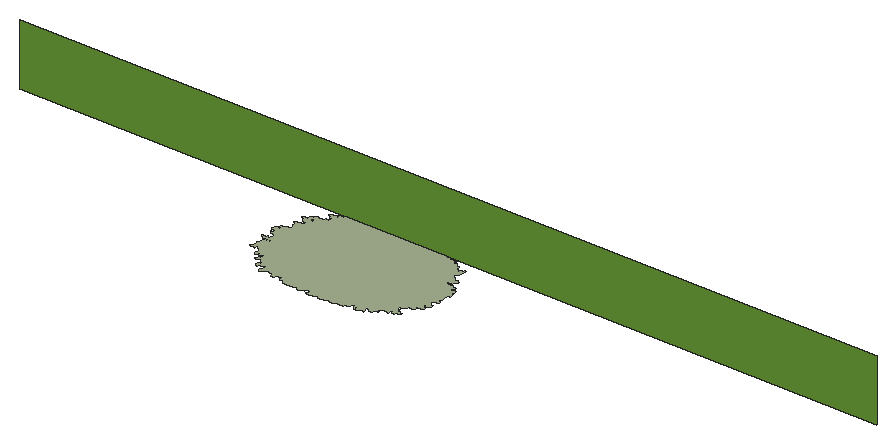
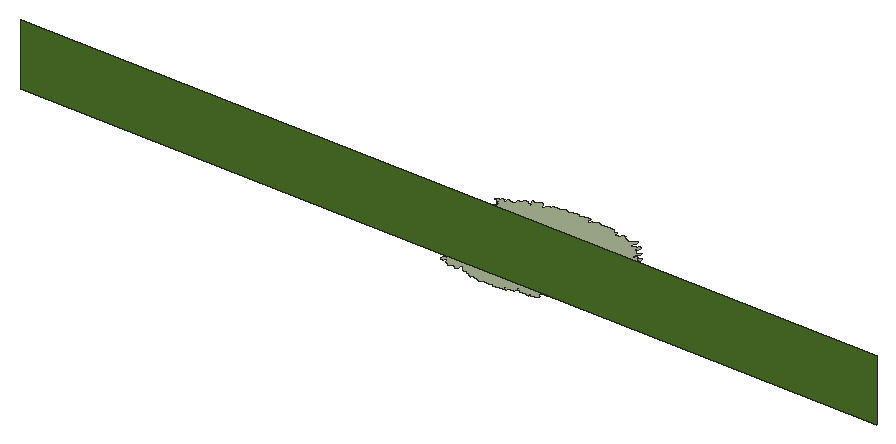
# SketchUp Ruby script. Lengths in inches.
U = 1.inch
M = Sketchup.active_model
def pt(a) = Geom::Point3d.new(a.map { |v| v * U })
def face(e, loops, mat)
  f = e.add_face(loops[0].map { |a| pt(a) })
  loops[1..].each { |l| e.add_face(l.map { |a| pt(a) }).erase! }
  f.material = f.back_material = mat if mat
  f
end
# faces: each face lists its corners as indices into pts; further lists are holes
def faces(e, pts, list, mat = nil) = list.each { |f| face(e, (f[0].is_a?(Array) ? f : [f]).map { |l| l.map { |i| pts[i] } }, mat) }
# xy, xz, yz: faces in a plane at the given z, y or x. An outline is a flat list of corners, or four numbers for a rectangle; further outlines are holes
def ring(l) = l.size == 4 ? [[l[0], l[1]], [l[2], l[1]], [l[2], l[3]], [l[0], l[3]]] : l.each_slice(2).to_a
def flat(e, list, mat, &to3) = list.each { |f| face(e, (f[0].is_a?(Array) ? f : [f]).map { |l| ring(l).map { |u, v| to3.(u, v) } }, mat) }
def xy(e, z, list, mat = nil) = flat(e, list, mat) { |x, y| [x, y, z] }
def xz(e, y, list, mat = nil) = flat(e, list, mat) { |x, z| [x, y, z] }
def yz(e, x, list, mat = nil) = flat(e, list, mat) { |y, z| [x, y, z] }
def lines(e, pts, list) = list.each { |a, b| e.add_line(pt(pts[a]), pt(pts[b])) }
# prism: a flat outline (further loops are holes) pulled along v
def prism(e, loops, v, mat = nil)
  f = face(e, loops, mat); d = Geom::Vector3d.new(v.map { |x| x * U })
  f.pushpull(f.normal.samedirection?(d) ? d.length : -d.length)
end
def box(e, o, s, mat = nil) = prism(e, [[o, [o[0] + s[0], o[1], o[2]], [o[0] + s[0], o[1] + s[1], o[2]], [o[0], o[1] + s[1], o[2]]]], [0, 0, s[2]], mat)
def at(x, y, z, deg = 0) = Geom::Transformation.translation(pt([x, y, z])) * Geom::Transformation.rotation(ORIGIN, Z_AXIS, deg.degrees)
def axes(o, x, y, z) = Geom::Transformation.new([*x, 0, *y, 0, *z, 0, *pt(o).to_a, 1])
def part(name) = M.definitions.add(name)
# library, detail: a bought-in or finely detailed component or shape, given as its bounding box
def library(name, o, s) = part(name).tap { |d| box(d.entities, o, s) }
def detail(e, o, s) = box(e.add_group.entities, o, s)
def put(e, d, t, mat = nil) = e.add_instance(d, t).tap { |i| i.material = mat if mat }
def group(e, t, mat = nil) = e.add_group.tap { |g| g.transformation = t; g.material = mat if mat }.entities
root = M.entities
M.materials.add("Boxwoodplan").color = [166, 177, 144]
M.materials.add("[Grass Dark Green]").color = [106, 157, 55]
xy(root,9.058,[[[87.354,67.129,87.243,67.133,87.148,67.159,87.092,67.215,87.091,67.317,87.117,67.382,87.18,67.445,87.229,67.509,87.288,67.606,87.101,67.635,87.011,67.644,87.031,67.732,87.117,67.79,87.148,67.8,87.143,67.846,87.054,67.877,86.938,67.837,86.841,67.706,86.699,67.551,86.538,67.464,86.432,67.441,86.372,67.416,86.356,67.373,86.211,67.281,86.018,67.251,85.929,67.26,85.848,67.306,85.848,67.328,85.894,67.359,85.984,67.437,86.053,67.483,85.963,67.498,85.851,67.48,85.731,67.436,85.537,67.454,85.44,67.447,85.314,67.403,85.113,67.356,85.024,67.349,84.986,67.443,84.978,67.465,84.911,67.473,84.822,67.454,84.654,67.336,84.454,67.328,84.224,67.353,84.057,67.446,83.915,67.61,84.098,67.702,83.999,67.756,83.863,67.772,83.737,67.749,83.664,67.697,83.584,67.672,83.468,67.738,83.426,67.806,83.513,67.847,83.54,67.907,83.545,67.957,83.504,68.009,83.431,68.085,83.346,68.117,83.259,68.064,83.192,68.038,83.136,68.08,83.12,68.103,83.096,68.121,83.066,68.111,82.987,68.058,82.915,68.01,82.839,67.923,82.828,67.79,82.756,67.749,82.706,67.723,82.646,67.725,82.547,67.746,82.461,67.793,82.417,67.861,82.408,67.951,82.417,68.018,82.43,68.04,82.411,68.08,82.198,68.1,82.266,68.135,82.239,68.136,82.147,68.13,81.977,68.146,81.9,68.173,81.883,68.206,81.897,68.224,82.023,68.314,82.02,68.371,81.936,68.393,81.776,68.39,81.646,68.319,81.548,68.233,81.474,68.199,81.426,68.172,81.425,68.154,81.462,68.101,81.446,68.046,81.375,68.081,81.312,68.121,81.251,68.072,81.228,68.017,81.197,67.904,81.149,67.855,81.076,67.822,80.985,67.816,80.915,67.841,80.897,67.874,80.904,67.892,80.925,67.932,80.947,67.991,80.916,68.048,80.815,68.149,80.929,68.229,80.99,68.269,81.069,68.285,81.137,68.315,81.192,68.37,81.276,68.476,81.205,68.503,81.125,68.511,80.993,68.53,80.954,68.565,80.962,68.584,81.036,68.62,81.198,68.657,81.241,68.709,81.236,68.748,81.21,68.764,81.06,68.711,81.014,68.732,81.015,68.752,81.037,68.814,80.876,68.825,80.796,68.833,80.742,68.826,80.734,68.806,80.718,68.71,80.703,68.642,80.662,68.591,80.615,68.578,80.595,68.594,80.536,68.639,80.492,68.757,80.452,68.783,80.425,68.784,80.372,68.777,80.365,68.757,80.363,68.641,80.308,68.523,80.248,68.449,80.168,68.419,80.089,68.422,80.042,68.448,80.009,68.506,80.01,68.564,80.063,68.677,80.177,68.784,80.198,68.803,80.184,68.823,80.158,68.829,80.077,68.847,79.997,68.86,79.97,68.875,79.976,68.895,79.997,68.914,80.145,68.982,80.307,69.005,80.349,69.108,80.323,69.169,80.276,69.191,80.248,69.187,80.085,69.168,80.045,69.2,80.051,69.22,80.079,69.279,80.236,69.334,80.408,69.403,80.457,69.442,80.443,69.463,80.347,69.436,80.175,69.417,80.031,69.372,79.942,69.386,79.915,69.392,79.922,69.412,79.942,69.426,79.997,69.47,79.97,69.507,79.942,69.503,79.86,69.511,79.805,69.56,79.791,69.601,79.763,69.597,79.681,69.575,79.524,69.489,79.374,69.413,79.3,69.38,79.245,69.392,79.258,69.412,79.278,69.452,79.304,69.469,79.329,69.55,79.378,69.65,79.41,69.759,79.461,69.812,79.535,69.852,79.579,69.972,79.601,70.112,79.62,70.227,79.616,70.285,79.571,70.321,79.491,70.335,79.404,70.335,79.331,70.31,79.321,70.245,79.321,70.184,79.288,70.124,79.2,70.087,79.144,70.096,79.105,70.155,79.095,70.216,79.069,70.337,79.063,70.4,79.023,70.453,78.995,70.475,78.958,70.491,78.899,70.479,78.864,70.46,78.863,70.428,78.855,70.366,78.857,70.229,78.882,70.167,78.874,70.103,78.824,70.038,78.775,70.01,78.737,69.998,78.7,70.003,78.658,70.011,78.64,70.039,78.636,70.166,78.657,70.223,78.702,70.276,78.718,70.306,78.709,70.334,78.652,70.34,78.571,70.346,78.533,70.362,78.51,70.39,78.507,70.453,78.523,70.483,78.557,70.499,78.73,70.472,78.808,70.497,78.858,70.526,78.918,70.573,78.932,70.636,78.909,70.662,78.865,70.664,78.787,70.67,78.695,70.681,78.594,70.717,78.576,70.746,78.581,70.76,78.601,70.763,78.66,70.775,78.836,70.761,78.925,70.787,78.938,70.844,78.912,70.907,78.84,70.946,78.761,70.953,78.647,70.946,78.548,70.921,78.464,70.939,78.46,70.968,78.481,70.997,78.527,71.054,78.594,71.11,78.647,71.19,78.638,71.224,78.594,71.241,78.529,71.24,78.411,71.14,78.371,71.141,78.337,71.161,78.358,71.22,78.375,71.287,78.331,71.35,78.291,71.366,78.271,71.367,78.266,71.352,78.27,71.306,78.267,71.164,78.226,71.102,78.186,71.108,78.152,71.131,78.054,71.262,78.029,71.327,78.005,71.355,77.989,71.344,77.934,71.293,77.899,71.234,77.918,71.103,77.923,71.037,77.903,70.971,77.854,70.962,77.819,70.978,77.809,71.023,77.829,71.155,77.839,71.233,77.839,71.27,77.824,71.282,77.809,71.272,77.729,71.237,77.69,71.183,77.68,71.12,77.641,71.077,77.504,70.987,77.465,70.977,77.42,70.986,77.341,71.026,77.32,71.056,77.324,71.089,77.357,71.151,77.455,71.237,77.544,71.263,77.634,71.263,77.729,71.267,77.669,71.318,77.517,71.404,77.501,71.466,77.554,71.503,77.645,71.573,77.764,71.635,77.883,71.709,77.918,71.723,77.944,71.746,77.971,71.789,77.974,71.882,78.006,72.003,78.007,72.065,77.986,72.086,77.965,72.095,77.902,72.109,77.868,72.104,77.865,72.088,77.876,71.996,77.835,71.934,77.787,71.899,77.709,71.871,77.638,71.858,77.478,71.833,77.443,71.839,77.429,71.853,77.43,71.86,77.438,71.901,77.455,71.947,77.497,71.995,77.567,72.042,77.625,72.063,77.684,72.065,77.722,72.068,77.742,72.075,77.765,72.096,77.761,72.121,77.706,72.151,77.638,72.207,77.606,72.264,77.602,72.331,77.615,72.382,77.668,72.426,77.694,72.432,77.705,72.425,77.724,72.411,77.767,72.35,77.816,72.304,77.945,72.226,78.018,72.192,78.054,72.177,78.074,72.184,78.098,72.206,78.104,72.222,78.116,72.263,78.1,72.32,78.058,72.366,78.025,72.389,77.992,72.401,77.932,72.401,77.858,72.404,77.814,72.446,77.728,72.519,77.67,72.569,77.631,72.617,77.631,72.646,77.655,72.671,77.712,72.698,77.747,72.703,77.788,72.7,77.848,72.679,77.909,72.677,77.945,72.684,77.98,72.726,78.028,72.757,78.088,72.764,78.159,72.764,78.3125,72.771,78.453,72.792,78.485,72.808,78.486,72.826,78.48,72.868,78.469,72.913,78.48,72.957,78.51,73.06,78.496,73.083,78.474,73.097,78.417,73.126,78.363,73.164,78.291,73.192,78.218,73.195,78.167,73.184,78.146,73.17,78.121,73.119,78.126,73.098,78.138,73.093,78.161,73.088,78.312,73.076,78.338,73.071,78.344,73.0625,78.334,73.046,78.295,73.007,78.249,72.964,78.185,72.928,78.123,72.884,78.05,72.849,78.013,72.852,77.994,72.863,77.968,72.9,77.961,72.995,77.944,73.02,77.962,73.034,77.969,73.077,77.963,73.088,77.951,73.088,77.937,73.087,77.911,73.083,77.878,73.076,77.861,73.065,77.78,72.97,77.748,72.915,77.717,72.892,77.694,72.895,77.668,72.916,77.659,72.932,77.653,72.973,77.681,73.057,77.687,73.102,77.678,73.13,77.657,73.137,77.619,73.128,77.599,73.114,77.553,73.064,77.432,72.957,77.395,72.932,77.37,72.927,77.332,72.935,77.32,72.951,77.412,73.057,77.474,73.102,77.488,73.129,77.488,73.145,77.479,73.152,77.467,73.148,77.453,73.143,77.421,73.131,77.338,73.108,77.17,73.089,77.097,73.096,77.05,73.121,77.028,73.149,77.027,73.165,77.044,73.217,77.091,73.264,77.152,73.281,77.222,73.284,77.297,73.266,77.424,73.223,77.51,73.197,77.522,73.201,77.522,73.209,77.521,73.22,77.512,73.239,77.488,73.287,77.486,73.342,77.494,73.407,77.505,73.437,77.523,73.45,77.571,73.413,77.611,73.363,77.638,73.317,77.647,73.255,77.66,73.204,77.674,73.176,77.698,73.175,77.832,73.157,77.905,73.144,77.94,73.14,77.958,73.154,77.974,73.202,77.918,73.244,77.86,73.309,77.842,73.335,77.842,73.352,77.876,73.46,77.906,73.483,77.934,73.489,77.948,73.477,77.957,73.459,77.986,73.414,77.998,73.39,78.01,73.391,78.031,73.404,78.111,73.482,78.127,73.528,78.129,73.579,78.115,73.611,78.094,73.623,78.03,73.646,77.991,73.666,77.982,73.687,77.998,73.736,78.054,73.773,78.089,73.795,78.102,73.816,78.109,73.869,78.108,73.916,78.012,73.992,77.869,74.014,77.806,74.031,77.772,74.013,77.743,74.014,77.674,74.031,77.655,74.058,77.665,74.082,77.791,74.185,77.784,74.217,77.762,74.233,77.718,74.225,77.689,74.216,77.563,74.154,77.523,74.107,77.473,74.063,77.404,74.049,77.376,74.05,77.329,74.102,77.357,74.126,77.375,74.165,77.407,74.188,77.5,74.22,77.545,74.25,77.535,74.281,77.522,74.283,77.512,74.276,77.486,74.27,77.446,74.273,77.311,74.284,77.165,74.3125,77.141,74.327,77.146,74.347,77.171,74.375,77.384,74.435,77.448,74.434,77.508,74.419,77.569,74.391,77.595,74.393,77.602,74.403,77.651,74.48,77.674,74.495,77.681,74.515,77.68,74.557,77.68,74.583,77.67,74.593,77.656,74.591,77.599,74.591,77.541,74.585,77.494,74.568,77.47,74.576,77.45,74.596,77.425,74.63,77.405,74.718,77.415,74.806,77.445,74.848,77.451,74.88,77.464,74.923,77.502,74.944,77.497,74.99,77.475,75.026,77.386,75.003,77.369,74.969,77.37,74.95,77.373,74.886,77.292,74.839,77.151,74.745,76.996,74.7,76.912,74.725,76.87,74.778,76.86,74.904,76.989,74.99,77.071,75.003,77.115,75.027,77.139,75.061,77.137,75.081,77.052,75.112,76.979,75.138,76.917,75.194,76.952,75.249,77.028,75.278,77.124,75.312,77.189,75.311,77.367,75.267,77.46,75.246,77.544,75.25,77.595,75.269,77.601,75.289,77.586,75.355,77.525,75.407,77.48,75.415,77.368,75.485,77.321,75.527,77.306,75.564,77.3,75.617,77.3,75.644,77.3125,75.659,77.355,75.695,77.406,75.709,77.52,75.741,77.55,75.751,77.591,75.75,77.641,75.746,77.653,75.733,77.668,75.703,77.683,75.689,77.692,75.689,77.721,75.692,77.737,75.704,77.757,75.754,77.785,75.787,77.802,75.81,77.804,75.835,77.821,75.86,77.84,75.872,77.888,75.884,77.927,75.877,77.949,75.833,77.953,75.781,77.969,75.755,77.991,75.754,78.032,75.796,78.057,75.838,78.072,75.942,78.087,75.968,78.12,75.975,78.151,75.974,78.171,75.963,78.192,75.94,78.224,75.94,78.276,75.961,78.321,76.007,78.335,76.032,78.324,76.046,78.384,76.043,78.413,76.046,78.428,76.066,78.433,76.114,78.467,76.155,78.502,76.2,78.448,76.243,78.38,76.272,78.343,76.271,78.311,76.261,78.268,76.249,78.227,76.255,78.205,76.271,78.183,76.295,78.16,76.397,78.173,76.423,78.179,76.439,78.189,76.443,78.293,76.463,78.339,76.472,78.358,76.483,78.348,76.486,78.262,76.514,78.196,76.526,78.168,76.519,78.132,76.52,78.096,76.52,78.061,76.532,78.022,76.582,78.004,76.611,78.004,76.642,78.02,76.663,78.049,76.678,78.08,76.697,78.088,76.725,78.118,76.782,78.145,76.836,78.151,76.89,78.143,76.917,78.103,76.928,78.025,76.954,77.852,77.001,77.817,77.018,77.8,77.042,77.835,77.097,77.88,77.131,77.925,77.159,77.98,77.178,78.033,77.1875,78.085,77.184,78.14,77.16,78.196,77.162,78.222,77.167,78.236,77.187,78.253,77.228,78.29,77.264,78.31,77.282,78.337,77.284,78.406,77.267,78.468,77.256,78.494,77.253,78.518,77.268,78.604,77.336,78.692,77.401,78.745,77.498,78.742,77.542,78.7,77.579,78.583,77.617,78.458,77.647,78.371,77.719,78.314,77.755,78.245,77.776,78.217,77.788,78.204,77.808,78.226,77.855,78.274,77.896,78.272,77.981,78.222,78.06,78.092,78.116,77.852,78.196,77.803,78.212,77.783,78.246,77.854,78.31,77.975,78.362,78.081,78.367,78.138,78.353,78.182,78.327,78.23,78.317,78.283,78.326,78.344,78.337,78.374,78.368,78.388,78.448,78.406,78.483,78.459,78.482,78.516,78.471,78.564,78.451,78.631,78.392,78.656,78.358,78.67,78.318,78.671,78.249,78.677,78.245,78.685,78.249,78.712,78.262,78.764,78.268,78.852,78.271,78.932,78.235,78.967,78.17,78.991,78.092,79.061,78.047,79.102,78.035,79.119,78.034,79.146,78.043,79.242,78.05,79.258,78.055,79.238,78.071,79.175,78.095,79.124,78.099,79.085,78.118,79.066,78.152,79.063,78.164,79.067,78.184,79.082,78.191,79.116,78.192,79.158,78.185,79.265,78.156,79.379,78.152,79.431,78.159,79.45,78.162,79.476,78.173,79.432,78.203,79.39,78.213,79.304,78.228,79.246,78.242,79.206,78.244,79.183,78.248,79.158,78.263,79.107,78.289,79.06,78.315,79.037,78.348,79.048,78.404,79.076,78.442,79.117,78.471,79.077,78.502,79.022,78.517,78.98,78.52,78.924,78.528,78.893,78.555,78.876,78.591,78.861,78.6,78.833,78.599,78.717,78.571,78.665,78.557,78.615,78.559,78.568,78.562,78.518,78.578,78.47,78.595,78.43,78.602,78.344,78.65,78.37,78.662,78.371,78.669,78.383,78.709,78.398,78.745,78.424,78.782,78.455,78.814,78.499,78.839,78.552,78.862,78.598,78.873,78.704,78.867,78.781,78.862,78.814,78.858,78.824,78.857,78.824,78.87,78.816,78.912,78.795,78.956,78.759,78.995,78.717,79.026,78.684,79.073,78.686,79.096,78.696,79.117,78.744,79.147,78.796,79.17,78.822,79.169,78.848,79.163,78.903,79.148,78.97,79.142,79.018,79.127,79.041,79.114,79.06,79.095,79.103,79.055,79.142,79.02,79.187,78.989,79.244,78.976,79.297,78.981,79.343,79.01,79.374,79.046,79.423,79.084,79.449,79.083,79.472,79.069,79.512,79.027,79.559,78.994,79.6875,79.019,79.762,79.037,79.803,79.065,79.809,79.085,79.787,79.102,79.736,79.124,79.727,79.147,79.735,79.169,79.75,79.214,79.757,79.273,79.761,79.299,79.784,79.315,79.812,79.316,79.842,79.308,79.884,79.288,80.018,79.248,80.078,79.226,80.118,79.193,80.144,79.153,80.159,79.13,80.166,79.123,80.176,79.126,80.184,79.131,80.216,79.176,80.222,79.212,80.212,79.315,80.191,79.362,80.167,79.397,80.131,79.436,80.121,79.466,80.133,79.477,80.144,79.475,80.165,79.476,80.165,79.484,80.17,79.508,80.162,79.549,80.148,79.705,80.15,79.782,80.034,79.802,79.937,79.804,79.875,79.8125,79.857,79.819,79.843,79.83,79.856,79.839,79.969,79.882,80.003,79.911,80.003,79.924,79.98,79.948,79.944,79.952,79.891,79.94,79.843,79.918,79.825,79.919,79.81,79.945,79.837,80.028,79.839,80.069,79.839,80.082,79.815,80.103,79.726,80.085,79.613,80.088,79.503,80.105,79.442,80.185,79.44,80.213,79.478,80.25,79.575,80.303,79.623,80.33,79.678,80.335,79.802,80.332,79.894,80.337,79.953,80.346,79.993,80.384,80.034,80.418,80.041,80.461,80.068,80.5,80.123,80.513,80.161,80.509,80.204,80.475,80.215,80.389,80.222,80.3,80.245,80.257,80.301,80.231,80.392,80.212,80.447,80.234,80.465,80.276,80.442,80.319,80.396,80.355,80.339,80.442,80.375,80.521,80.45,80.603,80.469,80.606,80.492,80.576,80.511,80.528,80.586,80.447,80.613,80.421,80.604,80.475,80.586,80.57,80.643,80.587,80.704,80.582,80.831,80.578,80.944,80.575,81.065,80.557,81.084,80.557,81.071,80.587,81.021,80.629,80.89,80.681,80.852,80.689,80.83,80.735,80.832,80.826,80.866,80.871,80.915,80.896,81.031,80.901,81.128,80.91,81.223,80.977,81.35,80.982,81.466,80.971,81.561,80.953,81.682,80.946,81.725,80.991,81.739,81.038,81.782,81.133,81.871,81.187,81.991,81.244,82.002,81.26,81.986,81.294,81.945,81.332,81.838,81.413,81.769,81.487,81.712,81.528,81.655,81.57,81.685,81.577,81.684,81.591,81.68,81.612,81.668,81.679,81.672,81.709,81.707,81.744,81.789,81.785,81.872,81.821,81.911,81.827,81.967,81.826,82.053,81.816,82.077,81.808,82.101,81.81,82.132,81.843,82.184,81.918,82.22,81.932,82.277,81.936,82.379,81.93,82.475,81.898,82.508,81.877,82.537,81.835,82.538,81.765,82.54,81.736,82.545,81.715,82.569,81.704,82.622,81.715,82.667,81.745,82.728,81.798,82.753,81.822,82.775,81.834,82.787,81.85,82.703,81.897,82.665,81.913,82.621,81.956,82.596,82.036,82.597,82.067,82.656,82.083,82.847,82.055,82.944,82.039,82.98,82.026,82.979,81.98,82.989,81.952,83.05,81.948,83.154,81.962,83.255,81.975,83.298,81.971,83.344,81.957,83.372,81.934,83.396,81.933,83.421,81.943,83.565,81.972,83.606,81.981,83.659,81.987,83.695,81.984,83.739,81.957,83.77,81.886,83.796,81.863,83.841,81.844,83.881,81.833,83.921,81.808,83.973,81.753,84.026,81.696,84.013,81.619,84.007,81.545,84.021,81.515,84.052,81.485,84.078,81.461,84.125,81.453,84.162,81.45,84.206,81.481,84.22,81.512,84.221,81.553,84.209,81.628,84.245,81.787,84.234,81.817,84.216,81.829,84.193,81.833,84.154,81.834,84.102,81.828,84.065,81.826,84.019,81.835,83.993,81.858,84.001,81.88,84.028,81.896,84.068,81.91,84.113,81.937,84.138,82.013,84.141,82.178,84.142,82.21,84.164,82.228,84.191,82.233,84.289,82.222,84.488,82.201,84.58,82.19,84.668,82.169,84.755,82.153,84.806,82.147,84.802,82.355,84.87,82.427,84.954,82.486,85.009,82.477,85.036,82.441,85.085,82.37,85.108,82.297,85.116,82.26,85.114,82.241,85.141,82.206,85.246,82.173,85.298,82.173,85.336,82.204,85.339,82.279,85.237,82.36,85.159,82.419,85.171,82.453,85.215,82.49,85.308,82.541,85.358,82.55,85.439,82.538,85.544,82.537,85.566,82.615,85.776,82.643,85.877,82.661,85.984,82.647,86.064,82.578,86.097,82.543,86.123,82.541,86.163,82.568,86.161,82.643,86.153,82.685,86.165,82.72,86.216,82.729,86.271,82.715,86.342,82.621,86.363,82.548,86.396,82.513,86.444,82.498,86.495,82.503,86.542,82.53,86.63,82.613,86.711,82.668,86.8125,82.715,86.861,82.7,86.874,82.663,86.823,82.592,86.797,82.557,86.805,82.515,86.893,82.457,86.993,82.443,87.044,82.452,87.093,82.498,87.172,82.566,87.286,82.581,87.401,82.553,87.433,82.523,87.509,82.492,87.61,82.511,87.691,82.565,87.691,82.678,87.749,82.721,87.862,82.745,87.967,82.74,88.048,82.681,88.194,82.66,88.247,82.651,88.253,82.614,88.18,82.546,88.147,82.473,88.159,82.437,88.23,82.396,88.333,82.401,88.385,82.433,88.405,82.472,88.426,82.544,88.474,82.567,88.498,82.579,88.55,82.579,88.653,82.541,88.696,82.47,88.781,82.417,88.912,82.447,88.946,82.478,88.953,82.52,88.992,82.603,89.099,82.622,89.129,82.592,89.135,82.55,89.083,82.466,89.034,82.448,89.007,82.413,89.068,82.349,89.198,82.337,89.289,82.373,89.357,82.444,89.381,82.45,89.39,82.433,89.409,82.392,89.433,82.357,89.421,82.301,89.402,82.257,89.42,82.222,89.509,82.179,89.617,82.184,89.672,82.203,89.722,82.258,89.739,82.273,89.742,82.255,89.728,82.212,89.656,82.132,89.622,82.102,89.633,82.066,89.68,82.047,89.737,82.048,89.834,82.088,89.916,82.146,90.136,82.225,90.157,82.153,90.18,82.123,90.232,82.118,90.347,82.11,90.471,82.084,90.486,82.013,90.509,81.983,90.556,81.964,90.579,81.93,90.564,81.892,90.538,81.795,90.654,81.773,90.7,81.755,90.711,81.72,90.637,81.65,90.622,81.613,90.639,81.579,90.714,81.527,90.818,81.5,90.919,81.496,91.031,81.563,91.073,81.639,91.015,81.71,90.982,81.779,91.002,81.885,91.011,81.922,90.982,81.956,90.978,81.992,91.019,82.018,91.12,82.022,91.109,82.122,91.068,82.274,91.117,82.287,91.182,82.275,91.235,82.256,91.267,82.199,91.217,82.131,91.22,82.095,91.267,82.076,91.375,82.076,91.504,82.111,92.012,82.178,92.057,82.168,92.103,82.145,92.15,82.121,92.184,82.097,92.215,82.027,92.197,81.935,92.402,81.949,92.467,81.943,92.551,81.911,92.588,81.805,92.574,81.757,92.557,81.724,92.516,81.717,92.347,81.749,92.282,81.755,92.24,81.755,92.219,81.749,92.216,81.733,92.245,81.685,92.285,81.666,92.333,81.666,92.505,81.681,92.574,81.683,92.659,81.648,92.696,81.609,92.726,81.546,92.794,81.437,92.874,81.398,92.958,81.394,92.989,81.435,92.983,81.518,92.965,81.571,92.972,81.637,93.013,81.687,93.115,81.719,93.224,81.732,93.3125,81.701,93.36,81.659,93.394,81.597,93.395,81.551,93.334,81.495,93.267,81.482,93.226,81.471,93.194,81.437,93.198,81.407,93.248,81.389,93.346,81.363,93.417,81.339,93.437,81.306,93.425,81.275,93.371,81.247,93.283,81.24,93.122,81.233,93.034,81.222,92.946,81.256,92.881,81.269,92.8,81.251,92.743,81.208,92.742,81.143,92.8,81.103,92.887,81.081,92.972,81.066,93.019,81.066,93.053,81.046,93.075,81.003,93.058,80.938,93.023,80.89,92.995,80.866,92.95,80.854,92.807,80.834,92.787,80.829,92.778,80.784,92.783,80.751,92.827,80.732,92.895,80.731,92.936,80.731,92.986,80.746,93.049,80.778,93.063,80.712,93.033,80.665,93.027,80.635,93.066,80.617,93.127,80.622,93.208,80.67,93.264,80.711,93.292,80.736,93.33,80.721,93.394,80.704,93.463,80.651,93.459,80.603,93.416,80.537,93.383,80.472,93.402,80.448,93.449,80.445,93.524,80.456,93.606,80.495,93.645,80.554,93.717,80.597,93.777,80.609,93.814,80.601,93.833,80.577,93.836,80.548,93.819,80.521,93.791,80.497,93.793,80.483,93.813,80.481,93.985,80.499,94.066,80.51,94.133,80.552,94.175,80.589,94.254,80.614,94.351,80.619,94.375,80.595,94.378,80.566,94.217,80.349,94.232,80.304,94.289,80.251,94.372,80.237,94.462,80.255,94.53,80.283,94.614,80.305,94.679,80.213,94.716,79.999,94.717,79.985,94.754,79.974,94.837,79.996,94.848,79.918,94.872,79.871,94.948,79.861,95.086,79.896,95.154,79.893,95.168,79.839,95.1,79.619,95.09,79.567,95.113,79.514,95.179,79.486,95.247,79.496,95.383,79.523,95.403,79.419,95.398,79.316,95.52,79.247,95.652,79.216,95.683,79.318,95.672,79.421,95.65,79.474,95.678,79.525,95.746,79.535,95.785,79.482,95.807,79.429,95.855,79.395,95.933,79.418,95.986,79.467,96.011,79.583,96.014,79.636,96.075,79.659,96.133,79.631,96.163,79.577,96.137,79.455,96.022,79.375,95.969,79.339,95.949,79.282,95.929,79.231,95.951,79.186,96.083,79.161,96.14,79.134,96.144,79.083,96.072,78.997,96.106,78.895,96.136,78.844,96.124,78.794,95.99,78.768,95.888,78.729,95.785,78.658,95.733,78.623,95.668,78.626,95.604,78.659,95.571,78.667,95.545,78.643,95.59,78.549,95.709,78.483,95.755,78.445,95.752,78.396,95.837,78.32,96.004,78.132,96.135,78.05,96.199,78.035,96.236,77.992,96.221,77.898,96.336,77.834,96.273,77.749,96.253,77.697,96.252,77.673,96.283,77.661,96.42,77.679,96.555,77.755,96.684,77.768,96.809,77.734,96.813,77.687,96.746,77.66,96.721,77.644,96.735,77.62,96.8125,77.599,96.884,77.596,96.916,77.595,96.93,77.571,96.841,77.482,96.675,77.322,96.651,77.232,96.647,77.187,96.62,77.142,96.526,77.067,96.398,77.038,96.273,77.043,96.165,77.082,96.095,77.076,96.068,77.004,96.096,76.894,96.066,76.787,95.948,76.72,95.976,76.62,96.114,76.642,96.286,76.833,96.514,76.815,96.59,76.605,96.635,76.595,96.716,76.618,96.804,76.723,96.942,76.735,96.979,76.635,96.929,76.574,96.915,76.539,96.991,76.501,97.13,76.531,97.25,76.598,97.297,76.614,97.386,76.592,97.364,76.477,97.254,76.384,97.189,76.289,97.196,76.113,97.182,76.078,97.09,76.056,96.957,76.087,96.982,75.981,97.114,75.941,97.26,75.936,97.408,75.965,97.645,76.087,97.782,76.099,97.874,76.008,97.841,75.905,97.701,75.849,97.653,75.825,97.625,75.766,97.728,75.675,97.879,75.515,97.847,75.414,97.73,75.359,97.694,75.335,97.733,75.274,97.876,75.269,98.007,75.247,98.018,75.145,97.946,75.089,97.812,75.078,97.687,75.041,97.644,74.942,97.8125,74.761,97.705,74.568,97.709,74.388,97.763,74.176,97.807,74.078,97.674,74.051,97.551,74.008,97.458,73.931,97.43,73.869,97.542,73.801,97.793,73.744,97.87,73.662,97.891,73.559,97.849,73.467,97.735,73.394,97.274,73.234,97.275,73.141,97.319,73.048,97.373,72.954,97.375,72.863,97.366,72.773,97.392,72.719,97.513,72.676,97.638,72.672,97.765,72.682,97.806,72.68,97.864,72.633,97.875,72.453,97.848,72.395,97.739,72.347,97.613,72.33,97.572,72.331,97.525,72.281,97.568,72.191,97.554,72.163,97.47,72.144,97.429,72.145,97.359,72.17,97.326,72.26,97.257,72.292,97.133,72.297,97.091,72.291,97.076,72.233,97.151,72.156,97.238,71.992,97.267,71.969,97.293,71.918,97.31,71.888,97.391,71.877,97.472,71.86,97.557,71.792,97.62,71.71,97.617,71.681,97.532,71.656,97.284,71.616,97.088,71.488,97.015,71.469,96.921,71.544,96.881,71.553,96.817,71.52,96.82,71.435,96.876,71.27,96.834,71.264,96.8,71.219,96.751,71.18,96.698,71.066,96.659,71.019,96.624,71,96.589,71.013,96.466,71.1,96.404,71.115,96.361,71.116,96.316,71.098,96.253,71.063,96.223,70.991,96.232,70.938,96.214,70.874,96.053,70.852,96,70.81,95.968,70.759,95.922,70.718,95.91,70.655,95.879,70.609,95.845,70.583,95.807,70.573,95.738,70.564,95.64,70.575,95.58,70.55,95.519,70.502,95.489,70.457,95.563,70.419,95.59,70.376,95.554,70.32,95.5,70.284,95.479,70.225,95.478,70.209,95.476,70.194,95.496,70.186,95.567,70.18,95.593,70.182,95.613,70.182,95.617,70.166,95.58,70.097,95.56,70.049,95.557,70.02,95.598,70.018,95.738,70.094,95.806,70.11,95.888,70.107,95.871,70.004,95.854,69.89,95.854,69.843,95.877,69.82,95.917,69.818,95.98,69.845,96.061,69.846,96.12,69.832,96.16,69.827,96.167,69.798,96.127,69.76,96.048,69.73,95.981,69.722,95.898,69.696,95.859,69.658,95.843,69.602,95.846,69.587,95.886,69.586,95.969,69.611,96.126,69.673,96.281,69.703,96.406,69.705,96.459,69.685,96.434,69.611,96.413,69.569,96.351,69.518,96.199,69.492,96.059,69.491,95.999,69.482,95.968,69.427,95.993,69.308,95.978,69.264,95.897,69.243,95.761,69.255,95.703,69.261,95.659,69.314,95.651,69.426,95.65,69.468,95.638,69.496,95.63,69.511,95.61,69.512,95.551,69.525,95.547,69.581,95.548,69.595,95.545,69.61,95.525,69.614,95.446,69.617,95.388,69.591,95.344,69.536,95.306,69.499,95.282,69.44,95.292,69.391,95.348,69.354,95.423,69.254,95.419,69.155,95.411,69.115,95.403,69.088,95.372,69.066,95.353,69.067,95.331,69.098,95.302,69.157,95.237,69.258,95.196,69.298,95.183,69.312,95.172,69.299,95.165,69.271,95.162,69.227,95.143,69.173,95.137,69.16,95.107,69.144,95.023,69.137,94.883,69.139,94.596,69.14,94.539,69.162,94.452,69.173,94.432,69.163,94.426,69.133,94.477,69.074,94.502,68.976,94.495,68.936,94.464,68.896,94.439,68.889,94.379,68.88,94.276,68.88,94.179,68.884,94.13,68.853,94.186,68.829,94.287,68.814,94.394,68.78,94.469,68.726,94.55,68.654,94.532,68.629,94.472,68.614,94.371,68.621,94.333,68.63,94.283,68.65,94.234,68.684,94.184,68.708,94.149,68.63,94.14,68.558,94.099,68.545,94.043,68.558,93.999,68.589,93.986,68.6,93.967,68.608,93.956,68.59,93.922,68.513,93.923,68.485,93.957,68.448,94.049,68.416,94.087,68.383,94.101,68.34,94.099,68.326,94.079,68.323,94.037,68.36,93.957,68.409,93.863,68.427,93.806,68.429,93.795,68.415,93.816,68.39,93.93,68.347,93.966,68.335,93.99,68.292,93.986,68.264,93.984,68.251,93.941,68.249,93.829,68.26,93.724,68.295,93.689,68.325,93.68,68.371,93.678,68.441,93.628,68.461,93.568,68.442,93.468,68.449,93.37,68.467,93.343,68.489,93.318,68.526,93.322,68.568,93.328,68.583,93.29,68.591,93.196,68.616,93.157,68.618,93.138,68.619,93.103,68.606,93.091,68.577,93.072,68.571,93.045,68.597,93.041,68.612,93.072,68.635,93.087,68.646,93.08,68.671,92.992,68.729,92.955,68.752,92.936,68.756,92.856,68.716,92.836,68.71,92.824,68.681,92.847,68.59,92.943,68.587,92.981,68.582,93.012,68.541,93.005,68.513,92.999,68.499,93.006,68.471,93.118,68.434,93.205,68.396,93.267,68.338,93.283,68.3125,93.282,68.299,93.248,68.283,93.228,68.273,93.259,68.251,93.313,68.225,93.325,68.2,93.275,68.168,93.263,68.141,93.288,68.106,93.373,68.062,93.45,67.994,93.45,67.851,93.428,67.825,93.376,67.814,93.322,67.829,93.285,67.874,93.244,67.939,93.227,67.949,93.189,67.944,93.136,67.926,93.115,67.897,93.116,67.854,93.115,67.84,93.081,67.828,92.905,67.819,92.896,67.826,92.849,67.808,92.805,67.777,92.721,67.692,92.668,67.661,92.595,67.651,92.457,67.643,92.403,67.658,92.4,67.698,92.509,67.762,92.61,67.834,92.607,67.937,92.6,67.98,92.601,67.994,92.569,68.015,92.51,68.034,92.435,68.034,92.352,67.95,92.332,67.911,92.274,67.866,92.26,67.857,92.223,67.865,92.187,67.88,92.174,67.907,92.215,67.999,92.274,68.094,92.276,68.135,92.208,68.189,92.096,68.224,92.045,68.246,92.007,68.238,91.983,68.215,91.949,68.171,91.916,68.156,91.874,68.157,91.818,68.166,91.78,68.168,91.742,68.145,91.662,68.05,91.675,68.01,91.749,67.97,91.804,67.938,91.832,67.917,91.841,67.89,91.817,67.851,91.756,67.807,91.655,67.756,91.599,67.735,91.526,67.738,91.471,67.76,91.398,67.769,91.352,67.745,91.316,67.743,91.284,67.76,91.229,67.766,91.156,67.752,91.133,67.717,91.144,67.659,91.24,67.575,91.268,67.536,91.268,67.497,91.25,67.492,90.961,67.391,90.685,67.369,90.452,67.373,90.362,67.371,90.239,67.31,90.136,67.275,90.039,67.279,90.002,67.281,89.952,67.299,89.904,67.328,89.844,67.325,89.755,67.334,89.671,67.376,89.611,67.433,89.579,67.478,89.521,67.491,89.421,67.479,89.326,67.438,89.245,67.398,89.146,67.325,89.049,67.269,88.956,67.24,88.715,67.222,88.525,67.186,88.429,67.19,88.364,67.284,88.333,67.351,88.244,67.365,88.153,67.352,88.057,67.28,87.992,67.217,87.902,67.21,87.726,67.233,87.54,67.24,87.462,67.189],[77.862,74.415,77.905,74.419,77.924,74.422,77.95,74.431,77.962,74.474,77.963,74.513,77.97,74.597,77.962,74.631,77.95,74.643,77.951,74.658,77.907,74.635,77.851,74.612,77.832,74.606,77.816,74.59,77.794,74.557,77.785,74.52,77.787,74.476,77.806,74.437,77.824,74.421]]],"Boxwoodplan")
xz(root,80.932,[[42.011,9,144.115,16.375]],"[Grass Dark Green]")
